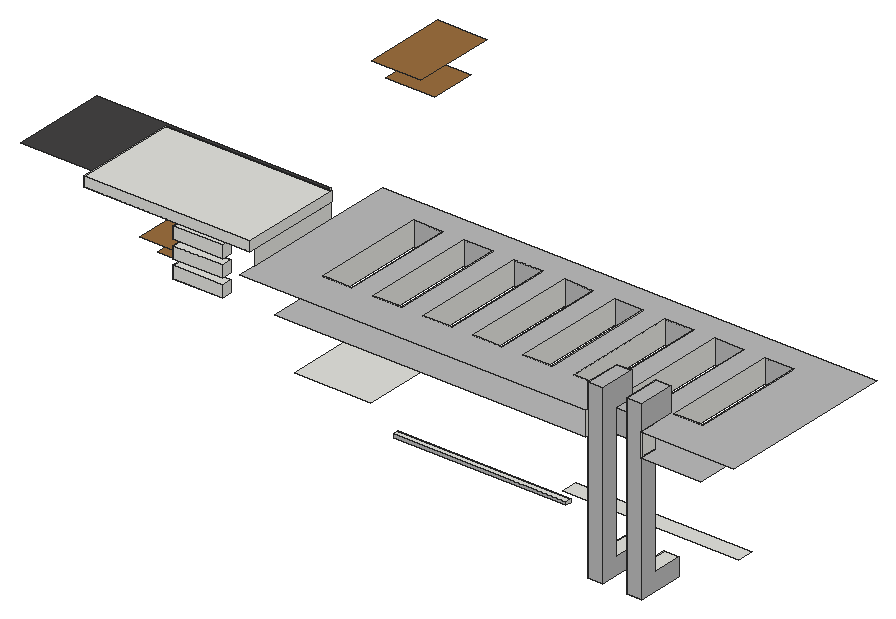
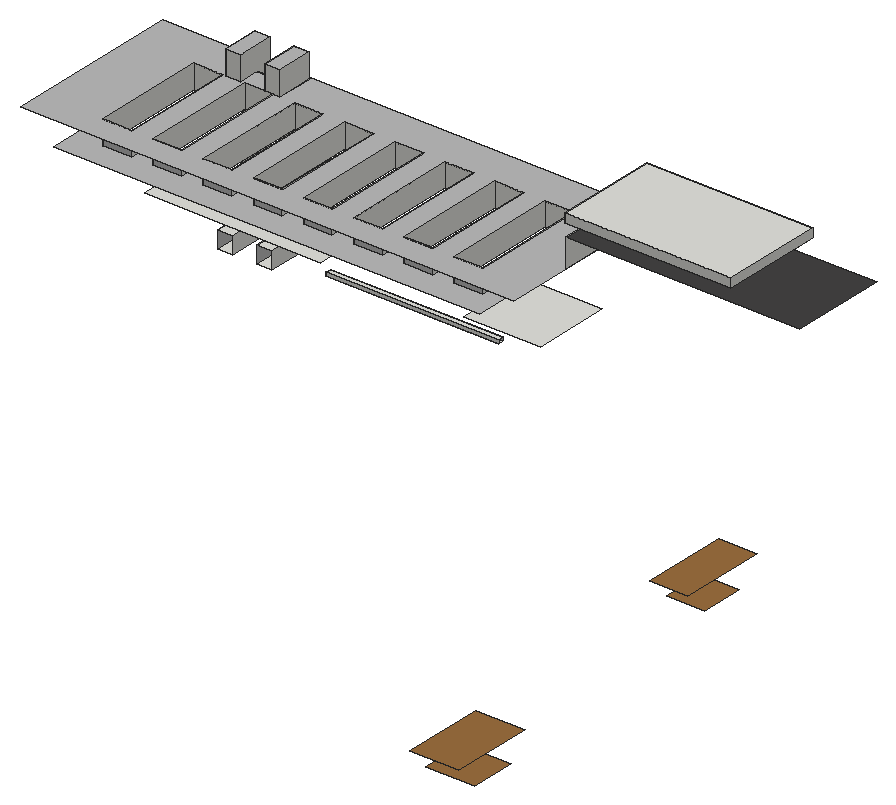
# SketchUp Ruby script. Lengths in inches.
U = 1.inch
M = Sketchup.active_model
def pt(a) = Geom::Point3d.new(a.map { |v| v * U })
def face(e, loops, mat)
  f = e.add_face(loops[0].map { |a| pt(a) })
  loops[1..].each { |l| e.add_face(l.map { |a| pt(a) }).erase! }
  f.material = f.back_material = mat if mat
  f
end
# faces: each face lists its corners as indices into pts; further lists are holes
def faces(e, pts, list, mat = nil) = list.each { |f| face(e, (f[0].is_a?(Array) ? f : [f]).map { |l| l.map { |i| pts[i] } }, mat) }
# xy, xz, yz: faces in a plane at the given z, y or x. An outline is a flat list of corners, or four numbers for a rectangle; further outlines are holes
def ring(l) = l.size == 4 ? [[l[0], l[1]], [l[2], l[1]], [l[2], l[3]], [l[0], l[3]]] : l.each_slice(2).to_a
def flat(e, list, mat, &to3) = list.each { |f| face(e, (f[0].is_a?(Array) ? f : [f]).map { |l| ring(l).map { |u, v| to3.(u, v) } }, mat) }
def xy(e, z, list, mat = nil) = flat(e, list, mat) { |x, y| [x, y, z] }
def xz(e, y, list, mat = nil) = flat(e, list, mat) { |x, z| [x, y, z] }
def yz(e, x, list, mat = nil) = flat(e, list, mat) { |y, z| [x, y, z] }
def lines(e, pts, list) = list.each { |a, b| e.add_line(pt(pts[a]), pt(pts[b])) }
# prism: a flat outline (further loops are holes) pulled along v
def prism(e, loops, v, mat = nil)
  f = face(e, loops, mat); d = Geom::Vector3d.new(v.map { |x| x * U })
  f.pushpull(f.normal.samedirection?(d) ? d.length : -d.length)
end
def box(e, o, s, mat = nil) = prism(e, [[o, [o[0] + s[0], o[1], o[2]], [o[0] + s[0], o[1] + s[1], o[2]], [o[0], o[1] + s[1], o[2]]]], [0, 0, s[2]], mat)
def at(x, y, z, deg = 0) = Geom::Transformation.translation(pt([x, y, z])) * Geom::Transformation.rotation(ORIGIN, Z_AXIS, deg.degrees)
def axes(o, x, y, z) = Geom::Transformation.new([*x, 0, *y, 0, *z, 0, *pt(o).to_a, 1])
def part(name) = M.definitions.add(name)
# library, detail: a bought-in or finely detailed component or shape, given as its bounding box
def library(name, o, s) = part(name).tap { |d| box(d.entities, o, s) }
def detail(e, o, s) = box(e.add_group.entities, o, s)
def put(e, d, t, mat = nil) = e.add_instance(d, t).tap { |i| i.material = mat if mat }
def group(e, t, mat = nil) = e.add_group.tap { |g| g.transformation = t; g.material = mat if mat }.entities
root = M.entities
M.materials.add("Generic").color = [155, 110, 63]
M.materials.add("Generic\#2").color = [186, 186, 186]
M.materials.add("[Granite Dark Gray]").color = [68, 67, 67]
box(root,[193.63,87.8125,1160.4],[44.69,9.4375,10.75])
box(root,[193.63,87.8125,1176.21],[44.69,9.4375,10.75])
box(root,[193.63,87.8125,1192.02],[44.69,9.4375,10.75])
xy(root,1046.8125,[[35,268.32,69,306.87],[4.375,563.94,48.5,603.53]],"Generic")
xy(root,1053.3125,[[570.42,82.8125,584.1,124.5],[605.79,82.8125,619.48,124.5]])
xy(root,1067.5625,[[35,249,69,326.1875],[4.375,547.73,48.5,621.86]],"Generic")
xy(root,1069,[[570.42,97.25,584.1,124.5],[605.79,97.25,619.48,124.5]])
xy(root,1072.38,[[[359.25,128.48,514.86,133.48],[366.79,129.75,367,129.78,367.2,129.86,367.37,129.99,367.5,130.16,367.58,130.36,367.61,130.57,367.58,130.78,367.5,130.97,367.37,131.14,367.2,131.27,367,131.35,366.79,131.38,366.58,131.35,366.39,131.27,366.22,131.14,366.09,130.97,366.01,130.78,365.98,130.57,366.01,130.36,366.09,130.16,366.22,129.99,366.39,129.86,366.58,129.78],[372.73,129.75,372.94,129.78,373.14,129.86,373.31,129.99,373.43,130.16,373.52,130.36,373.54,130.57,373.52,130.78,373.43,130.97,373.31,131.14,373.14,131.27,372.94,131.35,372.73,131.38,372.52,131.35,372.32,131.27,372.16,131.14,372.03,130.97,371.95,130.78,371.92,130.57,371.95,130.36,372.03,130.16,372.16,129.99,372.32,129.86,372.52,129.78],[378.98,129.75,379.19,129.78,379.39,129.86,379.56,129.99,379.68,130.16,379.77,130.36,379.79,130.57,379.77,130.78,379.68,130.97,379.56,131.14,379.39,131.27,379.19,131.35,378.98,131.38,378.77,131.35,378.57,131.27,378.41,131.14,378.28,130.97,378.2,130.78,378.17,130.57,378.2,130.36,378.28,130.16,378.41,129.99,378.57,129.86,378.77,129.78],[360.79,129.75,361,129.78,361.2,129.86,361.37,129.99,361.5,130.16,361.58,130.36,361.61,130.57,361.58,130.78,361.5,130.97,361.37,131.14,361.2,131.27,361,131.35,360.79,131.38,360.58,131.35,360.39,131.27,360.22,131.14,360.09,130.97,360.01,130.78,359.98,130.57,360.01,130.36,360.09,130.16,360.22,129.99,360.39,129.86,360.58,129.78],[385.23,129.75,385.44,129.78,385.64,129.86,385.81,129.99,385.93,130.16,386.02,130.36,386.04,130.57,386.02,130.78,385.93,130.97,385.81,131.14,385.64,131.27,385.44,131.35,385.23,131.38,385.02,131.35,384.82,131.27,384.66,131.14,384.53,130.97,384.45,130.78,384.42,130.57,384.45,130.36,384.53,130.16,384.66,129.99,384.82,129.86,385.02,129.78],[391.23,129.75,391.44,129.78,391.64,129.86,391.81,129.99,391.93,130.16,392.02,130.36,392.04,130.57,392.02,130.78,391.93,130.97,391.81,131.14,391.64,131.27,391.44,131.35,391.23,131.38,391.02,131.35,390.82,131.27,390.66,131.14,390.53,130.97,390.45,130.78,390.42,130.57,390.45,130.36,390.53,130.16,390.66,129.99,390.82,129.86,391.02,129.78],[397.54,129.75,397.75,129.78,397.95,129.86,398.12,129.99,398.25,130.16,398.33,130.36,398.36,130.57,398.33,130.78,398.25,130.97,398.12,131.14,397.95,131.27,397.75,131.35,397.54,131.38,397.33,131.35,397.14,131.27,396.97,131.14,396.84,130.97,396.76,130.78,396.73,130.57,396.76,130.36,396.84,130.16,396.97,129.99,397.14,129.86,397.33,129.78],[403.61,129.75,403.82,129.78,404.01,129.86,404.18,129.99,404.31,130.16,404.39,130.36,404.42,130.57,404.39,130.78,404.31,130.97,404.18,131.14,404.01,131.27,403.82,131.35,403.61,131.38,403.4,131.35,403.2,131.27,403.03,131.14,402.9,130.97,402.82,130.78,402.79,130.57,402.82,130.36,402.9,130.16,403.03,129.99,403.2,129.86,403.4,129.78],[409.73,129.75,409.94,129.78,410.14,129.86,410.31,129.99,410.43,130.16,410.52,130.36,410.54,130.57,410.52,130.78,410.43,130.97,410.31,131.14,410.14,131.27,409.94,131.35,409.73,131.38,409.52,131.35,409.32,131.27,409.16,131.14,409.03,130.97,408.95,130.78,408.92,130.57,408.95,130.36,409.03,130.16,409.16,129.99,409.32,129.86,409.52,129.78],[415.86,129.75,416.07,129.78,416.26,129.86,416.43,129.99,416.56,130.16,416.64,130.36,416.67,130.57,416.64,130.78,416.56,130.97,416.43,131.14,416.26,131.27,416.07,131.35,415.86,131.38,415.65,131.35,415.45,131.27,415.28,131.14,415.15,130.97,415.07,130.78,415.04,130.57,415.07,130.36,415.15,130.16,415.28,129.99,415.45,129.86,415.65,129.78],[421.98,129.75,422.19,129.78,422.39,129.86,422.56,129.99,422.68,130.16,422.77,130.36,422.79,130.57,422.77,130.78,422.68,130.97,422.56,131.14,422.39,131.27,422.19,131.35,421.98,131.38,421.77,131.35,421.57,131.27,421.41,131.14,421.28,130.97,421.2,130.78,421.17,130.57,421.2,130.36,421.28,130.16,421.41,129.99,421.57,129.86,421.77,129.78],[428.17,129.75,428.38,129.78,428.57,129.86,428.74,129.99,428.87,130.16,428.95,130.36,428.98,130.57,428.95,130.78,428.87,130.97,428.74,131.14,428.57,131.27,428.38,131.35,428.17,131.38,427.96,131.35,427.76,131.27,427.59,131.14,427.46,130.97,427.38,130.78,427.36,130.57,427.38,130.36,427.46,130.16,427.59,129.99,427.76,129.86,427.96,129.78],[434.23,129.75,434.44,129.78,434.64,129.86,434.81,129.99,434.93,130.16,435.02,130.36,435.04,130.57,435.02,130.78,434.93,130.97,434.81,131.14,434.64,131.27,434.44,131.35,434.23,131.38,434.02,131.35,433.82,131.27,433.66,131.14,433.53,130.97,433.45,130.78,433.42,130.57,433.45,130.36,433.53,130.16,433.66,129.99,433.82,129.86,434.02,129.78],[440.36,129.75,440.57,129.78,440.76,129.86,440.93,129.99,441.06,130.16,441.14,130.36,441.17,130.57,441.14,130.78,441.06,130.97,440.93,131.14,440.76,131.27,440.57,131.35,440.36,131.38,440.15,131.35,439.95,131.27,439.78,131.14,439.65,130.97,439.57,130.78,439.54,130.57,439.57,130.36,439.65,130.16,439.78,129.99,439.95,129.86,440.15,129.78],[446.36,129.75,446.57,129.78,446.76,129.86,446.93,129.99,447.06,130.16,447.14,130.36,447.17,130.57,447.14,130.78,447.06,130.97,446.93,131.14,446.76,131.27,446.57,131.35,446.36,131.38,446.15,131.35,445.95,131.27,445.78,131.14,445.65,130.97,445.57,130.78,445.54,130.57,445.57,130.36,445.65,130.16,445.78,129.99,445.95,129.86,446.15,129.78],[452.61,129.75,452.82,129.78,453.01,129.86,453.18,129.99,453.31,130.16,453.39,130.36,453.42,130.57,453.39,130.78,453.31,130.97,453.18,131.14,453.01,131.27,452.82,131.35,452.61,131.38,452.4,131.35,452.2,131.27,452.03,131.14,451.9,130.97,451.82,130.78,451.79,130.57,451.82,130.36,451.9,130.16,452.03,129.99,452.2,129.86,452.4,129.78],[458.54,129.75,458.75,129.78,458.95,129.86,459.12,129.99,459.25,130.16,459.33,130.36,459.36,130.57,459.33,130.78,459.25,130.97,459.12,131.14,458.95,131.27,458.75,131.35,458.54,131.38,458.33,131.35,458.14,131.27,457.97,131.14,457.84,130.97,457.76,130.78,457.73,130.57,457.76,130.36,457.84,130.16,457.97,129.99,458.14,129.86,458.33,129.78],[464.79,129.75,465,129.78,465.2,129.86,465.37,129.99,465.5,130.16,465.58,130.36,465.61,130.57,465.58,130.78,465.5,130.97,465.37,131.14,465.2,131.27,465,131.35,464.79,131.38,464.58,131.35,464.39,131.27,464.22,131.14,464.09,130.97,464.01,130.78,463.98,130.57,464.01,130.36,464.09,130.16,464.22,129.99,464.39,129.86,464.58,129.78],[471.17,129.75,471.38,129.78,471.57,129.86,471.74,129.99,471.87,130.16,471.95,130.36,471.98,130.57,471.95,130.78,471.87,130.97,471.74,131.14,471.57,131.27,471.38,131.35,471.17,131.38,470.96,131.35,470.76,131.27,470.59,131.14,470.46,130.97,470.38,130.78,470.36,130.57,470.38,130.36,470.46,130.16,470.59,129.99,470.76,129.86,470.96,129.78],[477.17,129.75,477.38,129.78,477.57,129.86,477.74,129.99,477.87,130.16,477.95,130.36,477.98,130.57,477.95,130.78,477.87,130.97,477.74,131.14,477.57,131.27,477.38,131.35,477.17,131.38,476.96,131.35,476.76,131.27,476.59,131.14,476.46,130.97,476.38,130.78,476.36,130.57,476.38,130.36,476.46,130.16,476.59,129.99,476.76,129.86,476.96,129.78],[483.23,129.75,483.44,129.78,483.64,129.86,483.81,129.99,483.93,130.16,484.02,130.36,484.04,130.57,484.02,130.78,483.93,130.97,483.81,131.14,483.64,131.27,483.44,131.35,483.23,131.38,483.02,131.35,482.82,131.27,482.66,131.14,482.53,130.97,482.45,130.78,482.42,130.57,482.45,130.36,482.53,130.16,482.66,129.99,482.82,129.86,483.02,129.78],[489.61,129.75,489.82,129.78,490.01,129.86,490.18,129.99,490.31,130.16,490.39,130.36,490.42,130.57,490.39,130.78,490.31,130.97,490.18,131.14,490.01,131.27,489.82,131.35,489.61,131.38,489.4,131.35,489.2,131.27,489.03,131.14,488.9,130.97,488.82,130.78,488.79,130.57,488.82,130.36,488.9,130.16,489.03,129.99,489.2,129.86,489.4,129.78],[495.61,129.75,495.82,129.78,496.01,129.86,496.18,129.99,496.31,130.16,496.39,130.36,496.42,130.57,496.39,130.78,496.31,130.97,496.18,131.14,496.01,131.27,495.82,131.35,495.61,131.38,495.4,131.35,495.2,131.27,495.03,131.14,494.9,130.97,494.82,130.78,494.79,130.57,494.82,130.36,494.9,130.16,495.03,129.99,495.2,129.86,495.4,129.78],[501.61,129.75,501.82,129.78,502.01,129.86,502.18,129.99,502.31,130.16,502.39,130.36,502.42,130.57,502.39,130.78,502.31,130.97,502.18,131.14,502.01,131.27,501.82,131.35,501.61,131.38,501.4,131.35,501.2,131.27,501.03,131.14,500.9,130.97,500.82,130.78,500.79,130.57,500.82,130.36,500.9,130.16,501.03,129.99,501.2,129.86,501.4,129.78],[507.61,129.75,507.82,129.78,508.01,129.86,508.18,129.99,508.31,130.16,508.39,130.36,508.42,130.57,508.39,130.78,508.31,130.97,508.18,131.14,508.01,131.27,507.82,131.35,507.61,131.38,507.4,131.35,507.2,131.27,507.03,131.14,506.9,130.97,506.82,130.78,506.79,130.57,506.82,130.36,506.9,130.16,507.03,129.99,507.2,129.86,507.4,129.78]]])
xy(root,1075.32,[[359.25,128.48,514.86,133.48]])
xy(root,1085.75,[[514.86,124.5,673.48,139.4375]])
xy(root,1111.375,[[290.4375,103.5,359.25,172.5]])
xy(root,1168.125,[[[290.4375,81.125,290.4375,241.25,673.48,241.25,673.48,81.125,619.48,81.125,619.48,97.25,570.42,97.25,570.42,81.125],[621.75,115.77,647.5625,218.39],[576.625,115.77,602.4375,218.39],[531.5,115.77,557.3125,218.39],[486.375,115.77,512.1875,218.39],[441.25,115.77,467.0625,218.39],[396.125,115.77,421.9375,218.39],[351,115.77,376.8125,218.39],[305.875,115.77,331.6875,218.39]]],"Generic\#2")
xy(root,1189.3125,[[570.42,97.25,584.1,115.77],[605.79,97.25,619.48,115.77]])
xy(root,1189.3125,[[[259.3125,81.125,570.42,81.125,570.42,115.77,576.625,115.77,576.625,218.39,602.4375,218.39,602.4375,115.77,584.1,115.77,584.1,97.25,605.79,97.25,605.79,115.77,619.48,115.77,619.48,81.125,703.6875,81.125,703.6875,241.25,259.3125,241.25],[621.75,115.77,647.5625,218.39],[531.5,115.77,557.3125,218.39],[486.375,115.77,512.1875,218.39],[441.25,115.77,467.0625,218.39],[396.125,115.77,421.9375,218.39],[351,115.77,376.8125,218.39],[305.875,115.77,331.6875,218.39]]],"Generic\#2")
xy(root,1211.125,[[570.42,82.8125,584.1,115.77],[605.79,82.8125,619.48,115.77]],"Generic\#2")
xy(root,1214.9375,[[123.04,75.875,259.3125,97.25],[259.3125,75.875,272.1875,167.57],[123.04,97.25,259.3125,167.57]])
xy(root,1214.9375,[[48.5,97.25,123.04,97.25,123.04,167.57,259.3125,167.57,259.3125,183.25,48.5,183.25]],"[Granite Dark Gray]")
xy(root,1223.3125,[[123.04,75.875,272.1875,167.57]])
xz(root,75.875,[[123.04,1214.9375,272.1875,1223.3125]])
xz(root,82.8125,[[570.42,1053.3125,584.1,1211.125],[605.79,1053.3125,619.48,1211.125]],"Generic\#2")
xz(root,97.25,[[570.42,1069,584.1,1168.125],[605.79,1069,619.48,1168.125],[570.42,1168.125,584.1,1189.3125],[605.79,1168.125,619.48,1189.3125]])
xz(root,97.25,[[584.1,1168.125,605.79,1189.3125]],"Generic\#2")
xz(root,115.77,[[305.875,1168.125,331.6875,1189.3125],[351,1168.125,376.8125,1189.3125],[396.125,1168.125,421.9375,1189.3125],[441.25,1168.125,467.0625,1189.3125],[486.375,1168.125,512.1875,1189.3125],
  [531.5,1168.125,557.3125,1189.3125],[576.625,1168.125,602.4375,1189.3125],[621.75,1168.125,647.5625,1189.3125],[570.42,1189.3125,584.1,1211.125],[605.79,1189.3125,619.48,1211.125]])
xz(root,128.48,[[359.25,1072.38,514.86,1075.32]],"Generic\#2")
xz(root,133.48,[[359.25,1072.38,514.86,1075.32]])
xz(root,167.57,[[123.04,1214.9375,272.1875,1223.3125]])
xz(root,218.39,[[305.875,1168.125,331.6875,1189.3125],[351,1168.125,376.8125,1189.3125],[396.125,1168.125,421.9375,1189.3125],[441.25,1168.125,467.0625,1189.3125],[486.375,1168.125,512.1875,1189.3125],
  [531.5,1168.125,557.3125,1189.3125],[576.625,1168.125,602.4375,1189.3125],[621.75,1168.125,647.5625,1189.3125]],"Generic\#2")
yz(root,123.04,[[75.875,1214.9375,167.57,1223.3125]])
yz(root,259.3125,[[97.25,1189.3125,183.25,1214.9375]])
yz(root,272.1875,[[75.875,1214.9375,167.57,1223.3125]])
yz(root,305.875,[[115.77,1168.125,218.39,1189.3125]])
yz(root,331.6875,[[115.77,1168.125,218.39,1189.3125]])
yz(root,351,[[115.77,1168.125,218.39,1189.3125]])
yz(root,376.8125,[[115.77,1168.125,218.39,1189.3125]])
yz(root,396.125,[[115.77,1168.125,218.39,1189.3125]])
yz(root,421.9375,[[115.77,1168.125,218.39,1189.3125]])
yz(root,441.25,[[115.77,1168.125,218.39,1189.3125]])
yz(root,467.0625,[[115.77,1168.125,218.39,1189.3125]])
yz(root,486.375,[[115.77,1168.125,218.39,1189.3125]])
yz(root,512.1875,[[115.77,1168.125,218.39,1189.3125]])
yz(root,514.86,[[128.48,1072.38,133.48,1075.32]])
yz(root,531.5,[[115.77,1168.125,218.39,1189.3125]])
yz(root,557.3125,[[115.77,1168.125,218.39,1189.3125]])
yz(root,570.42,[[82.8125,1053.3125,82.8125,1168.125,97.25,1168.125,97.25,1069,124.5,1069,124.5,1053.3125],[81.125,1168.125,82.8125,1189.3125],[82.8125,1168.125,97.25,1189.3125],[82.8125,1189.3125,115.77,1211.125]])
yz(root,576.625,[[115.77,1168.125,218.39,1189.3125]])
yz(root,584.1,[[82.8125,1053.3125,124.5,1053.3125,124.5,1069,97.25,1069,97.25,1189.3125,115.77,1189.3125,115.77,1211.125,82.8125,1211.125]],"Generic\#2")
yz(root,602.4375,[[115.77,1168.125,218.39,1189.3125]])
yz(root,605.79,[[82.8125,1053.3125,82.8125,1211.125,115.77,1211.125,115.77,1189.3125,97.25,1189.3125,97.25,1069,124.5,1069,124.5,1053.3125]])
yz(root,619.48,[[81.125,1168.125,82.8125,1189.3125],[82.8125,1168.125,97.25,1189.3125]])
yz(root,619.48,[[82.8125,1053.3125,124.5,1053.3125,124.5,1069,97.25,1069,97.25,1168.125,82.8125,1168.125],[82.8125,1189.3125,115.77,1211.125]],"Generic\#2")
yz(root,621.75,[[115.77,1168.125,218.39,1189.3125]])
yz(root,647.5625,[[115.77,1168.125,218.39,1189.3125]])
p = [[514.86,130.98,1073.97],[359.25,130.98,1073.97]]
lines(root,p,[[0,1]])
